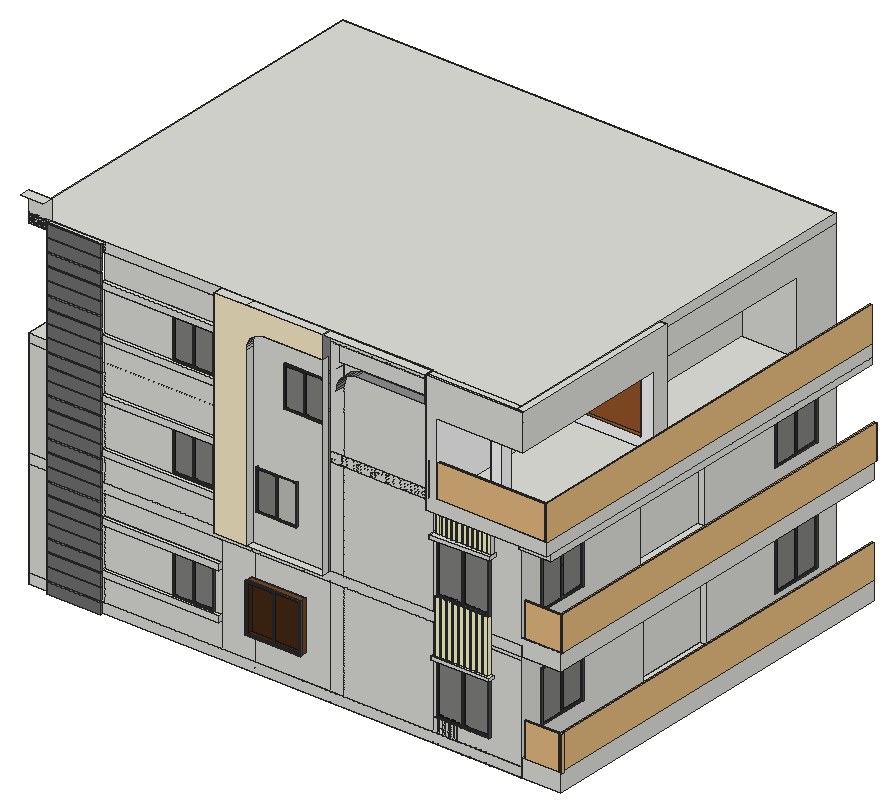
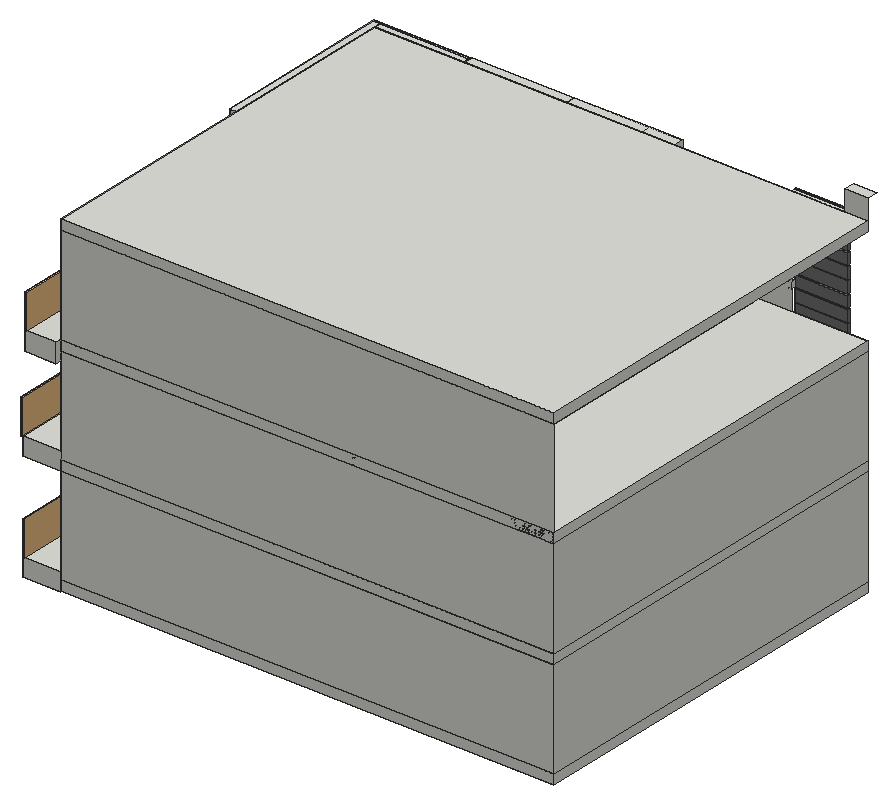
# SketchUp Ruby script. Lengths in inches.
U = 1.inch
M = Sketchup.active_model
def pt(a) = Geom::Point3d.new(a.map { |v| v * U })
def face(e, loops, mat)
  f = e.add_face(loops[0].map { |a| pt(a) })
  loops[1..].each { |l| e.add_face(l.map { |a| pt(a) }).erase! }
  f.material = f.back_material = mat if mat
  f
end
# faces: each face lists its corners as indices into pts; further lists are holes
def faces(e, pts, list, mat = nil) = list.each { |f| face(e, (f[0].is_a?(Array) ? f : [f]).map { |l| l.map { |i| pts[i] } }, mat) }
# xy, xz, yz: faces in a plane at the given z, y or x. An outline is a flat list of corners, or four numbers for a rectangle; further outlines are holes
def ring(l) = l.size == 4 ? [[l[0], l[1]], [l[2], l[1]], [l[2], l[3]], [l[0], l[3]]] : l.each_slice(2).to_a
def flat(e, list, mat, &to3) = list.each { |f| face(e, (f[0].is_a?(Array) ? f : [f]).map { |l| ring(l).map { |u, v| to3.(u, v) } }, mat) }
def xy(e, z, list, mat = nil) = flat(e, list, mat) { |x, y| [x, y, z] }
def xz(e, y, list, mat = nil) = flat(e, list, mat) { |x, z| [x, y, z] }
def yz(e, x, list, mat = nil) = flat(e, list, mat) { |y, z| [x, y, z] }
def lines(e, pts, list) = list.each { |a, b| e.add_line(pt(pts[a]), pt(pts[b])) }
# prism: a flat outline (further loops are holes) pulled along v
def prism(e, loops, v, mat = nil)
  f = face(e, loops, mat); d = Geom::Vector3d.new(v.map { |x| x * U })
  f.pushpull(f.normal.samedirection?(d) ? d.length : -d.length)
end
def box(e, o, s, mat = nil) = prism(e, [[o, [o[0] + s[0], o[1], o[2]], [o[0] + s[0], o[1] + s[1], o[2]], [o[0], o[1] + s[1], o[2]]]], [0, 0, s[2]], mat)
def at(x, y, z, deg = 0) = Geom::Transformation.translation(pt([x, y, z])) * Geom::Transformation.rotation(ORIGIN, Z_AXIS, deg.degrees)
def axes(o, x, y, z) = Geom::Transformation.new([*x, 0, *y, 0, *z, 0, *pt(o).to_a, 1])
def part(name) = M.definitions.add(name)
# library, detail: a bought-in or finely detailed component or shape, given as its bounding box
def library(name, o, s) = part(name).tap { |d| box(d.entities, o, s) }
def detail(e, o, s) = box(e.add_group.entities, o, s)
def put(e, d, t, mat = nil) = e.add_instance(d, t).tap { |i| i.material = mat if mat }
def group(e, t, mat = nil) = e.add_group.tap { |g| g.transformation = t; g.material = mat if mat }.entities
root = M.entities
M.materials.add("Glass_Tinted_Gray").color = [0, 0, 0]
M.materials["Glass_Tinted_Gray"].alpha = 0.125
M.materials.add("[0135_DarkGray]").color = [81, 81, 81]
M.materials.add("[Color D01]").color = [255, 242, 204]
M.materials.add("[Color E01]").color = [255, 255, 204]
M.materials.add("[Color M00]").color = [255, 255, 255]
M.materials.add("[Color M04]").color = [142, 142, 142]
M.materials.add("[Color M05]").color = [114, 114, 114]
M.materials.add("[Mirror 02]").color = [229, 229, 229]
M.materials.add("[Terrazzo Light Blue]").color = [196, 214, 227]
M.materials.add("[Wood Cherry Original]").color = [152, 86, 42]
M.materials.add("[Wood Veneer 01]").color = [120, 70, 37]
c1 = part("Group\#9")
box(c1.entities,[0,-2.75,0],[65.625,2.75,13.9375])
c2 = library("Wagner Glass Railing",[9.08,102.375,1.53],[2.51,145.5,42.05])
c3 = part("PENTEK_RP Fineline 50S_Sliding_DoorCase_E1")
box(c3.entities,[0,0,0],[1.51,3.66,99.27],"[0135_DarkGray]")
c4 = part("PENTEK_RP Fineline 50S_SlidingDooe_Case_E2")
box(c4.entities,[0,0,0],[96.25,3.66,1.51],"[0135_DarkGray]")
c5 = part("pentek_RP Fineline 50S_SlidingDoor_Case")
put(c5.entities,c3,at(97.76,0,0))
put(c5.entities,c4,at(1.51,0,0))
put(c5.entities,c3,at(0,0,0))
put(c5.entities,c4,at(1.51,0,97.76))
c6 = part("PENTEK_RP Fineline 50S_SlidingDoor_GlazingBead_2")
box(c6.entities,[0,0,0],[0.56,0.59,94.39],"[0135_DarkGray]")
c7 = part("PENTEK_RP Fineline 50S_SlidingDoor_Glass")
box(c7.entities,[0,0,0],[46.58,0.16,94.39],"Glass_Tinted_Gray")
c8 = part("PENTEK_RP Fineline 50S_SlidingDoor_GlazingBead")
box(c8.entities,[0,0,0],[45.47,0.59,0.56],"[0135_DarkGray]")
c9 = part("PENTEK_RP Fineline 50S_SlidingDoor_Leaf_E1")
xy(c9.entities,0,[[0,0,0.93,1.97],[0.93,1.57,1.49,1.97]],"[0135_DarkGray]")
xy(c9.entities,96.25,[[0,0,0.93,0,0.93,1.57,1.49,1.57,1.49,1.97,0,1.97]],"[0135_DarkGray]")
xz(c9.entities,0,[[0,0,0.93,96.25]],"[0135_DarkGray]")
xz(c9.entities,1.57,[[0.93,0,1.49,95.32],[0.93,95.32,1.49,96.25]],"[0135_DarkGray]")
xz(c9.entities,1.97,[[0,0,1.49,96.25]],"[0135_DarkGray]")
yz(c9.entities,0,[[0,0,1.97,96.25]],"[0135_DarkGray]")
yz(c9.entities,0.93,[[0,0,1.57,0.93],[0,0.93,1.57,95.32],[0,95.32,1.57,96.25]],"[0135_DarkGray]")
yz(c9.entities,1.49,[[1.57,0,1.97,95.32],[1.57,95.32,1.97,96.25]],"[0135_DarkGray]")
c10 = part("PENTEK_RP Fineline 50S_SlidingDoor_Leaf_E2")
xy(c10.entities,0,[[0,0,0,1.57,0.56,1.57,0.56,1.97,46.02,1.97,46.02,1.57,46.58,1.57,46.58,0]],"[0135_DarkGray]")
xy(c10.entities,0.93,[[0,0,46.58,1.57]],"[0135_DarkGray]")
xy(c10.entities,1.49,[[0.56,1.57,46.02,1.97]],"[0135_DarkGray]")
xz(c10.entities,0,[[0,0,46.58,0.93]],"[0135_DarkGray]")
xz(c10.entities,1.57,[[0,0,0.56,0.93],[46.02,0,46.58,0.93],[0.56,0.93,46.02,1.49]],"[0135_DarkGray]")
xz(c10.entities,1.97,[[0.56,0,46.02,1.49]],"[0135_DarkGray]")
yz(c10.entities,0,[[0,0,1.57,0.93]],"[0135_DarkGray]")
yz(c10.entities,0.56,[[1.57,0,1.97,0.93],[1.57,0.93,1.97,1.49]],"[0135_DarkGray]")
yz(c10.entities,46.02,[[1.57,0,1.97,0.93],[1.57,0.93,1.97,1.49]],"[0135_DarkGray]")
yz(c10.entities,46.58,[[0,0,1.57,0.93]],"[0135_DarkGray]")
c11 = part("PENTEK_RP Fineline S_SlidingDoor_Leaf1")
put(c11.entities,c6,at(0.93,0,0.93))
put(c11.entities,c6,at(46.96,0,0.93))
put(c11.entities,c7,at(1.49,1.42,0.93))
put(c11.entities,c8,at(1.49,0,0.93))
put(c11.entities,c7,at(1.49,0.59,0.93),"[Terrazzo Light Blue]")
put(c11.entities,c9,at(0,0,0))
put(c11.entities,c9,axes([48.44,0,0],[-1,0,0],[0,1,0],[0,0,1]))
put(c11.entities,c10,axes([0.93,0,96.25],[1,0,0],[0,1,0],[0,0,-1]))
put(c11.entities,c10,at(0.93,0,0))
put(c11.entities,c8,at(1.49,0,94.77))
c12 = part("PENTEK_RP Fineline 50S_SlidingDoor_Leaf2")
put(c12.entities,c7,at(1.49,1.42,0.93))
put(c12.entities,c8,at(1.49,0,94.77))
put(c12.entities,c6,at(46.96,0,0.93))
put(c12.entities,c7,at(1.49,0.59,0.93),"[Mirror 02]")
put(c12.entities,c6,at(0.93,0,0.93))
put(c12.entities,c9,at(0,0,0))
put(c12.entities,c9,axes([48.44,0,0],[-1,0,0],[0,1,0],[0,0,1]))
put(c12.entities,c8,at(1.49,0,0.93))
put(c12.entities,c10,axes([0.93,0,96.25],[1,0,0],[0,1,0],[0,0,-1]))
put(c12.entities,c10,at(0.93,0,0))
c13 = part("PENTEK - Slimmest Steel Sliding Door / Window\#1")
put(c13.entities,c5,at(0,-1.88,-0.09))
put(c13.entities,c11,at(1.51,-2.27,1.42))
put(c13.entities,c12,at(49.32,-0.3,1.42))
c14 = part("Group\#10")
box(c14.entities,[-76.71,-4.875,-2.4375],[142.83,4.875,7.6875])
prism(root,[[[538.49,59.34,350.59],[610.93,62.6,350.59],[611.36,53.02,350.59],[538.92,49.75,350.59]]],[0,0,4.15])
xy(root,119.69,[[643.25,62.39,690.1875,542.39]])
xy(root,120,[[[39.25,62.39,643.25,542.39],[172.25,71.39,634.25,533.39]]])
xy(root,132,[[[39.25,62.39,643.25,542.39],[172.25,71.39,634.25,533.39]],[172.25,71.39,634.25,533.39]])
xy(root,141.25,[[643.25,62.39,690.1875,542.39],[634.375,246.18,643.25,344.71]])
xy(root,152.27,[[540.39,57.14,545.76,62.39],[546.71,57.14,552.08,62.39],[553.03,57.14,558.4,62.39],[559.28,57.14,564.65,62.39],[565.65,57.14,571.03,62.39],
  [572.84,57.14,578.21,62.39],[579.65,57.14,585.03,62.39],[586.71,57.14,592.09,62.39],[592.73,57.14,598.11,62.39],[599.11,57.14,606.05,62.39]])
xy(root,165.75,[[313.83,50.27,379.89,59.77]],"[Wood Veneer 01]")
xy(root,216.35,[[538.15,53.52,608.9,62.39]])
xy(root,218.67,[[548.22,57.14,554.35,62.39],[555.28,57.14,561.41,62.39]])
xy(root,219.92,[[538.15,53.52,608.9,53.52,608.9,62.39,561.41,62.39,561.41,57.14,555.28,57.14,555.28,62.39,554.35,62.39,554.35,57.14,548.22,57.14,548.22,62.39,547.1,62.39,547.1,57.14,540.97,57.14,540.97,62.39,538.15,62.39]])
xy(root,225.5,[[313.83,50.27,379.89,59.77]],"[Wood Veneer 01]")
xy(root,252,[[[39.25,62.39,643.25,62.39,643.25,246.18,634.375,246.18,634.375,344.71,643.25,344.71,643.25,542.39,39.25,542.39],[172.25,71.39,634.25,533.39]],[643.25,62.39,643.25,246.18,634.375,246.18,634.375,344.71,643.25,344.71,643.25,542.39,690.1875,542.39,690.1875,62.39]])
xy(root,264,[[275.5,50.27,315.25,62.39],[315.25,50.27,408.24,59.45],[315.25,59.45,408.24,62.39],[172.25,71.39,634.25,533.39]])
xy(root,273.5625,[[643.25,62.39,690.1875,62.39,690.1875,542.39,643.25,542.39,643.25,341.58,634.375,341.58,634.375,242.52,643.25,242.52]])
xy(root,285.55,[[598.15,57.66,604.28,62.91]])
xy(root,285.71,[[540.97,57.14,547.1,62.39],[548.22,57.14,554.35,62.39],[555.28,57.14,561.41,62.39]])
xy(root,285.87,[[562.53,57.66,568.65,62.91],[569.46,57.66,575.59,62.91],[576.53,57.66,582.65,62.91],[584.03,57.66,590.15,62.91],[591.28,57.66,597.4,62.91]])
xy(root,351.625,[[541.21,57.14,546.27,62.39]])
xy(root,372.625,[[643.25,57.6,681.9,549.14],[634.375,242.52,643.25,272.93],[634.375,272.93,643.25,341.58]])
xy(root,379.8125,[[534.125,51.64,534.125,57.14,539.4375,57.14,539.4375,62.39,541.21,62.39,541.21,57.14,547.02,57.14,547.02,62.39,548.46,62.39,548.46,57.14,553.52,57.14,553.52,62.39,555.16,62.39,555.16,57.14,560.23,57.14,560.23,62.39,561.35,62.39,561.35,57.14,566.41,57.14,566.41,62.39,567.85,62.39,567.85,57.14,572.91,57.14,572.91,62.39,574.79,62.39,574.79,57.14,579.85,57.14,579.85,62.39,580.73,62.39,580.73,57.14,585.79,57.14,585.79,62.39,586.85,62.39,586.85,57.14,591.91,57.14,591.91,62.39,592.54,62.39,592.54,57.14,597.6,57.14,597.6,62.39,598.48,62.39,598.48,57.14,603.54,57.14,603.54,62.39,603.5625,62.39,603.5625,57.14,608.625,57.14,608.625,62.39,643.25,62.39,643.25,57.6,681.9,57.6,681.9,51.64],[534.125,57.14,539.4375,62.39],[541.21,57.14,546.27,62.39],[546.27,57.14,547.02,62.39],[548.46,57.14,553.52,62.39],
  [555.16,57.14,560.23,62.39],[561.35,57.14,566.41,62.39],[567.85,57.14,572.91,62.39],[574.79,57.14,579.85,62.39],[580.73,57.14,585.79,62.39],
  [586.85,57.14,591.91,62.39],[592.54,57.14,597.6,62.39],[598.48,57.14,603.54,62.39],[603.5625,57.14,608.625,62.39]])
xy(root,384,[[547.02,62.39,643.25,62.39,643.25,482.24,634.25,482.24,634.25,71.39,547.02,71.39]])
xy(root,396,[[547.02,51.64,681.9,51.64,681.9,272.93,652.0625,272.93,652.0625,252.8,643.25,252.8,643.25,62.39,547.02,62.39],[172.25,71.39,547.02,71.39,547.02,252.8,634.25,252.8,634.25,272.93,575.75,272.93,575.75,482.24,634.25,482.24,634.25,533.39,172.25,533.39],[634.25,252.8,643.25,272.93],[643.25,272.93,681.9,549.14]])
xy(root,396,[[592.44,78.38,605,93.32]],"[Wood Cherry Original]")
xy(root,407.63,[[565.8,252.8,635.55,258.68]],"[Wood Cherry Original]")
xy(root,470.57,[[565.8,252.8,635.55,258.68]],"[Wood Cherry Original]")
xy(root,480.375,[[[556.7,64.84,639.52,239.78],[592.44,78.38,605,93.32]],[584.07,281.12,632.51,473.74]],"[Wood Cherry Original]")
xy(root,484.0625,[[[547.02,51.64,652.0625,252.8],[556.7,64.84,639.52,239.78]],[[575.75,272.93,643.25,482.24],[584.07,281.12,632.51,473.74]]])
xy(root,496.9375,[[425.1875,62.39,449.88,64.02]])
xy(root,496.9375,[[449.88,50.27,533.5,62.39]],"[Color M04]")
xy(root,501.33,[[337.14,50.27,408.24,59.45]])
xy(root,516,[[[39.25,62.39,643.25,542.39],[172.25,71.39,634.25,533.39]]])
xy(root,528,[[275.5,50.27,315.25,62.39],[315.25,50.27,408.24,62.39],[408.24,50.27,533.5,62.39],[534.125,51.64,652.0625,53.64],[534.125,53.64,643.25,62.39],
  [643.25,53.64,652.0625,272.93],[67.04,57.77,132.66,62.39]])
xy(root,552.6875,[[39.25,49.27,67.04,62.39]])
xz(root,50.27,[[275.5,264,315.25,264,315.25,479.4375,315.4375,482.29,315.99,485.1,316.92,487.8125,318.18,490.38,319.77,492.76,321.66,494.92,323.8125,496.8,326.19,498.39,328.76,499.66,331.47,500.58,334.28,501.14,337.14,501.33,408.24,501.33,408.24,528,275.5,528]],"[Color D01]")
xz(root,51.64,[[534.125,379.8125,681.9,379.8125,681.9,396,547.02,396,547.02,484.0625,652.0625,484.0625,652.0625,528,534.125,528]])
xz(root,53.52,[[538.15,216.35,608.9,219.92]])
xz(root,57.14,[[548.22,218.67,554.35,219.92],[555.28,218.67,561.41,219.92]])
xz(root,57.14,[[540.97,219.92,547.1,285.71],[548.22,219.92,554.35,285.71],[555.28,219.92,561.41,285.71],[541.21,351.625,546.27,379.8125],[548.46,351.625,553.52,379.8125],
  [555.16,351.625,560.23,379.8125],[561.35,351.625,566.41,379.8125],[567.85,351.625,572.91,379.8125],[574.79,351.625,579.85,379.8125],[580.73,351.625,585.79,379.8125],
  [586.85,351.625,591.91,379.8125],[592.54,351.625,597.6,379.8125],[598.48,351.625,603.54,379.8125],[603.5625,351.625,608.625,379.8125]],"[Color E01]")
xz(root,57.6,[[643.25,372.625,681.9,379.8125]])
xz(root,57.66,[[562.53,216.45,568.65,285.87],[569.46,216.45,575.59,285.87],[576.53,216.45,582.65,285.87],[584.03,216.45,590.15,285.87],[591.28,216.45,597.4,285.87],
  [598.15,216.45,604.28,285.55]],"[Color E01]")
xz(root,59.45,[[315.25,264,408.24,264,408.24,501.33,337.14,501.33,334.28,501.14,331.47,500.58,328.76,499.66,326.19,498.39,323.8125,496.8,321.66,494.92,319.77,492.76,318.18,490.38,316.92,487.8125,315.99,485.1,315.4375,482.29,315.25,479.4375]])
xz(root,59.77,[[313.83,165.75,379.89,225.5]],"[Wood Veneer 01]")
xz(root,62.39,[[599.11,119.69,606.05,119.69,606.05,132,643.25,132,643.25,247.5,554.35,247.5,554.35,219.92,555.28,219.92,555.28,218.67,561.41,218.67,561.41,219.92,608.9,219.92,608.9,216.35,539.4375,216.35,539.4375,132,540.39,132,540.39,131.69,540.97,131.69,540.97,132,540.39,132,540.39,152.27,540.97,152.27,540.97,153.4,547.1,153.4,547.1,152.27,548.22,152.27,548.22,153.4,554.35,153.4,554.35,152.27,555.28,152.27,555.28,153.4,561.41,153.4,561.41,152.27,564.65,152.27,564.65,120,599.11,120],[561.41,119.69,564.65,120],[564.65,119.69,565.65,120],[565.65,119.69,571.03,120],[571.03,119.69,572.84,120],
  [572.84,119.69,578.21,120],[578.21,119.69,579.65,120],[579.65,119.69,585.03,120],[585.03,119.69,586.71,120],[586.71,119.69,592.09,120],
  [592.09,119.69,592.73,120],[592.73,119.69,598.11,120],[598.11,119.69,599.11,120],[599.11,119.69,606.05,120],[606.05,119.69,643.25,120],
  [643.25,119.69,690.1875,119.69,690.1875,141.25,643.25,141.25,643.25,132,606.05,132,606.05,120,643.25,120],[39.25,120,67.04,132],[67.04,120,132.66,132],[275.5,120,315.25,132],[315.25,120,408.24,132],
  [408.24,120,425.1875,132],[534.125,120,539.4375,132],[540.39,120,540.39,131.69,540.97,131.69,540.97,132,545.76,132,545.76,120],[561.41,120,564.65,132],[604.48,120,606.05,132],
  [539.4375,131.69,540.39,132],[547.1,131.69,548.22,132],[554.35,131.69,555.28,132],[39.25,132,67.04,252],[67.04,132,132.66,252],
  [132.66,132,275.5,252],[275.5,132,315.25,252],[315.25,132,408.24,252],[408.24,132,425.1875,252],[425.1875,132,534.125,252],
  [534.125,132,539.4375,132,539.4375,216.35,538.15,216.35,538.15,219.92,539.4375,219.92,539.4375,252,534.125,252],[539.4375,132,540.39,132,540.39,152.27,540.97,152.27,540.97,153.4,547.1,153.4,547.1,152.27,548.22,152.27,548.22,153.4,554.35,153.4,554.35,152.27,555.28,152.27,555.28,153.4,561.41,153.4,561.41,152.27,564.65,152.27,564.65,132,565.65,132,565.65,152.27,571.03,152.27,571.03,132,572.84,132,572.84,152.27,578.21,152.27,578.21,132,579.65,132,579.65,152.27,585.03,152.27,585.03,132,586.71,132,586.71,152.27,592.09,152.27,592.09,132,592.73,132,592.73,152.27,598.11,152.27,598.11,132,599.11,132,599.11,152.27,606.05,152.27,606.05,132,643.25,132,643.25,247.5,561.41,247.5,561.41,219.92,608.9,219.92,608.9,216.35,539.4375,216.35],[540.39,132,540.97,152.27],[545.76,132,546.71,132,546.71,152.27,547.1,152.27,547.1,153.4,540.97,153.4,540.97,152.27,545.76,152.27],[546.71,132,547.1,152.27],
  [547.1,132,548.22,152.27],[548.22,132,552.08,152.27],[552.08,132,553.03,132,553.03,152.27,554.35,152.27,554.35,153.4,548.22,153.4,548.22,152.27,552.08,152.27],[553.03,132,554.35,152.27],[554.35,132,555.28,152.27],
  [555.28,132,558.4,152.27],[558.4,132,559.28,132,559.28,152.27,561.41,152.27,561.41,153.4,555.28,153.4,555.28,152.27,558.4,152.27],[559.28,132,561.41,152.27],[561.41,132,564.65,152.27],[565.65,132,571.03,152.27],
  [572.84,132,578.21,152.27],[579.65,132,585.03,152.27],[586.71,132,592.09,152.27],[592.73,132,598.11,152.27],[599.11,132,606.05,152.27],
  [538.15,216.35,539.4375,219.92],[539.4375,216.35,608.9,216.35,608.9,219.92,561.41,219.92,561.41,218.67,555.28,218.67,555.28,219.92,554.35,219.92,554.35,218.67,548.22,218.67,548.22,219.92,547.1,219.92,547.1,218.67,540.97,218.67,540.97,219.92,539.4375,219.92],[540.97,218.67,547.1,218.67,547.1,247.5,546.27,247.5,546.27,219.32,541.21,219.32,541.21,247.5,540.97,247.5],[548.22,218.67,554.35,247.5],[555.28,218.67,561.41,247.5],
  [541.21,219.32,546.27,219.32,546.27,247.5,547.1,247.5,547.1,252,540.97,252,540.97,247.5,541.21,247.5],[539.4375,219.92,540.97,247.5],[547.1,219.92,548.22,247.5],[554.35,219.92,555.28,247.5],[539.4375,247.5,540.97,252],
  [547.1,247.5,548.22,252],[548.22,247.5,554.35,252],[554.35,247.5,555.28,252],[555.28,247.5,561.41,252],[561.41,247.5,643.25,252],
  [39.25,252,67.04,264],[67.04,252,132.66,264],[275.5,252,315.25,264],[315.25,252,408.24,264],[408.24,252,425.1875,264],
  [534.125,252,539.4375,264],[561.41,252,690.1875,252,690.1875,273.5625,643.25,273.5625,643.25,379.8125,546.27,379.8125,546.27,351.625,541.21,351.625,541.21,379.8125,539.4375,379.8125,539.4375,264,540.97,264,540.97,285.71,547.1,285.71,547.1,264,548.22,264,548.22,285.71,554.35,285.71,554.35,264,555.28,264,555.28,285.71,561.41,285.71],[540.97,252,547.1,259.125],[540.97,259.125,547.1,264],[39.25,264,67.04,384],
  [67.04,264,132.66,384],[132.66,264,275.5,264,275.5,481.34,209.375,481.34,209.375,486.59,275.5,486.59,275.5,516,132.66,516],[275.5,264,315.25,384],[315.25,264,408.24,384],[408.24,264,425.1875,384],
  [425.1875,264,534.125,384],[548.22,264,554.35,285.71],[555.28,264,561.41,285.71],[534.125,379.8125,547.02,384],[547.02,379.8125,643.25,384],
  [275.5,384,315.25,516],[315.25,384,408.24,516],[408.24,384,425.1875,384,425.1875,496.9375,418.125,496.9375,418.125,516,408.24,516],[425.1875,384,534.125,384,534.125,516,533.5,516,533.5,496.9375,533.61,496.9375,533.61,471.875,532.42,471.875,532.42,496.9375,425.1875,496.9375],[547.02,384,643.25,396],
  [418.125,496.9375,533.5,516],[39.25,516,67.04,552.6875],[67.04,516,132.66,528],[275.5,516,315.25,528],[315.25,516,408.24,528],
  [408.24,516,533.5,528],[534.125,516,643.25,528]])
xz(root,64.02,[[425.1875,472.24,425.1875,496.9375,449.88,496.9375,446.66,496.73,443.49,496.1,440.43,495.06,437.53,493.63,434.85,491.83,432.42,489.71,430.29,487.28,428.5,484.59,427.07,481.69,426.03,478.64,425.4,475.47]])
xz(root,64.84,[[556.7,480.375,639.52,484.0625]],"[Wood Cherry Original]")
xz(root,71.39,[[172.25,132,634.25,252],[172.25,264,634.25,384],[172.25,384,547.02,396]])
xz(root,78.38,[[592.44,396,605,480.375]],"[Color M00]")
xz(root,93.32,[[592.44,396,605,480.375]],"[Color M00]")
xz(root,239.78,[[556.7,480.375,639.52,484.0625]],"[Wood Cherry Original]")
xz(root,242.52,[[634.375,273.5625,643.25,372.625]])
xz(root,246.18,[[634.375,141.25,643.25,252]])
xz(root,252.8,[[[547.02,396,652.0625,484.0625],[565.8,407.63,635.55,470.57]]],"[Color M00]")
xz(root,258.68,[[565.8,407.63,635.55,470.57]],"[Wood Cherry Original]")
xz(root,272.93,[[575.75,396,643.25,484.0625],[643.25,396,652.0625,528]])
xz(root,281.12,[[584.07,480.375,632.51,484.0625]],"[Wood Cherry Original]")
xz(root,341.58,[[634.375,273.5625,643.25,372.625]])
xz(root,344.71,[[634.375,141.25,643.25,252]])
xz(root,473.74,[[584.07,480.375,632.51,484.0625]],"[Wood Cherry Original]")
xz(root,482.24,[[634.25,384,643.25,384,643.25,484.0625,575.75,484.0625,575.75,396,634.25,396]])
xz(root,533.39,[[172.25,132,634.25,252],[172.25,264,634.25,384],[172.25,384,634.25,396],[172.25,396,634.25,516]])
xz(root,542.39,[[643.25,119.69,690.1875,141.25],[39.25,132,643.25,252],[643.25,252,690.1875,273.5625],[39.25,264,643.25,384],[39.25,384,643.25,516]])
xz(root,549.14,[[643.25,372.625,681.9,396]])
yz(root,39.25,[[62.39,132,542.39,252],[62.39,264,542.39,384]])
yz(root,172.25,[[71.39,132,533.39,252],[71.39,264,533.39,384],[71.39,384,533.39,396],[71.39,396,533.39,516]])
yz(root,275.5,[[50.27,264,62.39,528]])
yz(root,313.83,[[50.27,165.75,59.77,225.5]],"[Wood Veneer 01]")
yz(root,315.25,[[50.27,264,59.45,479.4375]])
yz(root,379.89,[[50.27,165.75,59.77,225.5]],"[Wood Veneer 01]")
yz(root,408.24,[[50.27,264,59.45,501.33]])
yz(root,408.24,[[59.45,264,59.45,501.33,50.27,501.33,50.27,528,62.39,528,62.39,264]],"[Color M04]")
yz(root,425.1875,[[62.39,472.24,64.02,496.9375]])
yz(root,533.5,[[50.27,496.9375,62.39,528]],"[Color M04]")
yz(root,534.125,[[51.64,379.8125,62.39,516],[51.64,516,53.64,528],[53.64,516,62.39,528]])
yz(root,538.15,[[53.52,216.35,62.39,219.92]])
yz(root,540.97,[[57.14,219.92,62.39,285.71]])
yz(root,541.21,[[57.14,351.625,62.39,379.8125]],"[Color E01]")
yz(root,546.27,[[57.14,351.625,62.39,379.8125]],"[Color E01]")
yz(root,547.02,[[62.39,384,62.39,396,51.64,396,51.64,484.0625,252.8,484.0625,252.8,396,71.39,396,71.39,384]],"[Color M00]")
yz(root,547.1,[[57.14,219.92,62.39,285.71]],"[Color E01]")
yz(root,548.22,[[57.14,218.67,62.39,219.92],[57.14,219.92,62.39,285.71]])
yz(root,548.46,[[57.14,351.625,62.39,379.8125]],"[Color E01]")
yz(root,553.52,[[57.14,351.625,62.39,379.8125]],"[Color E01]")
yz(root,554.35,[[57.14,218.67,62.39,219.92]])
yz(root,554.35,[[57.14,219.92,62.39,285.71]],"[Color E01]")
yz(root,555.16,[[57.14,351.625,62.39,379.8125]],"[Color E01]")
yz(root,555.28,[[57.14,218.67,62.39,219.92],[57.14,219.92,62.39,285.71]])
yz(root,556.7,[[64.84,480.375,239.78,484.0625]],"[Wood Cherry Original]")
yz(root,560.23,[[57.14,351.625,62.39,379.8125]],"[Color E01]")
yz(root,561.35,[[57.14,351.625,62.39,379.8125]],"[Color E01]")
yz(root,561.41,[[57.14,218.67,62.39,219.92]])
yz(root,561.41,[[57.14,219.92,62.39,285.71]],"[Color E01]")
yz(root,562.53,[[57.66,216.45,62.91,285.87]])
yz(root,565.8,[[252.8,407.63,258.68,470.57]],"[Wood Cherry Original]")
yz(root,566.41,[[57.14,351.625,62.39,379.8125]],"[Color E01]")
yz(root,567.85,[[57.14,351.625,62.39,379.8125]],"[Color E01]")
yz(root,568.65,[[57.66,216.45,62.91,285.87]])
yz(root,569.46,[[57.66,216.45,62.91,285.87]])
yz(root,572.91,[[57.14,351.625,62.39,379.8125]],"[Color E01]")
yz(root,574.79,[[57.14,351.625,62.39,379.8125]],"[Color E01]")
yz(root,575.59,[[57.66,216.45,62.91,285.87]],"[Color E01]")
yz(root,575.75,[[272.93,396,482.24,484.0625]])
yz(root,576.53,[[57.66,216.45,62.91,285.87]])
yz(root,579.85,[[57.14,351.625,62.39,379.8125]],"[Color E01]")
yz(root,580.73,[[57.14,351.625,62.39,379.8125]],"[Color E01]")
yz(root,582.65,[[57.66,216.45,62.91,285.87]],"[Color E01]")
yz(root,584.03,[[57.66,216.45,62.91,285.87]])
yz(root,584.07,[[281.12,480.375,473.74,484.0625]])
yz(root,585.79,[[57.14,351.625,62.39,379.8125]],"[Color E01]")
yz(root,586.85,[[57.14,351.625,62.39,379.8125]],"[Color E01]")
yz(root,590.15,[[57.66,216.45,62.91,285.87]],"[Color E01]")
yz(root,591.28,[[57.66,216.45,62.91,285.87]])
yz(root,591.91,[[57.14,351.625,62.39,379.8125]],"[Color E01]")
yz(root,592.44,[[78.38,396,93.32,480.375]],"[Color M00]")
yz(root,592.54,[[57.14,351.625,62.39,379.8125]])
yz(root,597.4,[[57.66,216.45,62.91,285.87]],"[Color E01]")
yz(root,597.6,[[57.14,351.625,62.39,379.8125]],"[Color E01]")
yz(root,598.15,[[57.66,216.45,62.91,285.55]])
yz(root,598.48,[[57.14,351.625,62.39,379.8125]],"[Color E01]")
yz(root,603.54,[[57.14,351.625,62.39,379.8125]])
yz(root,603.5625,[[57.14,351.625,62.39,379.8125]])
yz(root,604.28,[[57.66,216.45,62.91,285.55]],"[Color E01]")
yz(root,605,[[78.38,396,93.32,480.375]],"[Color M00]")
yz(root,608.625,[[57.14,351.625,62.39,379.8125]])
yz(root,608.9,[[53.52,216.35,62.39,219.92]])
yz(root,632.51,[[281.12,480.375,473.74,484.0625]],"[Wood Cherry Original]")
yz(root,634.25,[[71.39,132,533.39,252],[71.39,264,533.39,384],[482.24,384,533.39,396]])
yz(root,634.375,[[246.18,141.25,344.71,252],[242.52,273.5625,341.58,372.625]])
yz(root,635.55,[[252.8,407.63,258.68,470.57]],"[Wood Cherry Original]")
yz(root,639.52,[[64.84,480.375,239.78,484.0625]],"[Wood Cherry Original]")
yz(root,643.25,[[62.39,119.69,542.39,120],[62.39,132,542.39,141.25],[62.39,141.25,246.18,252],[344.71,141.25,542.39,252],[62.39,273.5625,242.52,372.625],
  [341.58,273.5625,542.39,372.625],[57.6,372.625,62.39,379.8125],[62.39,372.625,272.93,384],[272.93,372.625,542.39,384],[542.39,372.625,549.14,396],
  [62.39,384,272.93,396],[272.93,384,482.24,396],[482.24,384,542.39,396],[482.24,396,542.39,396,542.39,516,272.93,516,272.93,484.0625,482.24,484.0625],[53.64,516,62.39,528],
  [62.39,516,272.93,528]])
yz(root,652.0625,[[252.8,396,272.93,396,272.93,528,51.64,528,51.64,484.0625,252.8,484.0625]])
yz(root,681.9,[[57.6,372.625,549.14,379.8125],[51.64,379.8125,549.14,396]])
yz(root,690.1875,[[62.39,119.69,542.39,141.25],[62.39,252,542.39,273.5625]])
p = [[425.4,50.27,475.47],[425.1875,50.27,472.24],[425.1875,62.39,472.24],[425.1875,64.02,472.24],[425.4,64.02,475.47],[426.03,50.27,478.64],
  [426.03,64.02,478.64],[427.07,50.27,481.69],[427.07,64.02,481.69],[315.4375,50.27,482.29],[315.25,50.27,479.4375],[315.25,59.45,479.4375],
  [315.4375,59.45,482.29],[428.5,50.27,484.59],[428.5,64.02,484.59],[315.99,50.27,485.1],[315.99,59.45,485.1],[430.29,50.27,487.28],
  [430.29,64.02,487.28],[316.92,50.27,487.8125],[316.92,59.45,487.8125],[432.42,50.27,489.71],[432.42,64.02,489.71],[318.18,50.27,490.38],
  [318.18,59.45,490.38],[434.85,50.27,491.83],[434.85,64.02,491.83],[319.77,50.27,492.76],[319.77,59.45,492.76],[437.53,50.27,493.63],
  [437.53,64.02,493.63],[321.66,50.27,494.92],[321.66,59.45,494.92],[440.43,50.27,495.06],[440.43,64.02,495.06],[323.8125,50.27,496.8],
  [323.8125,59.45,496.8],[443.49,50.27,496.1],[443.49,64.02,496.1],[446.66,50.27,496.73],[446.66,64.02,496.73],[449.88,50.27,496.9375],
  [449.88,64.02,496.9375],[449.88,62.39,496.9375],[326.19,50.27,498.39],[326.19,59.45,498.39],[328.76,50.27,499.66],[328.76,59.45,499.66],
  [331.47,50.27,500.58],[331.47,59.45,500.58],[334.28,50.27,501.14],[334.28,59.45,501.14],[337.14,50.27,501.33],[337.14,59.45,501.33],
  [425.1875,50.27,496.9375],[425.1875,62.39,496.9375],[634.25,71.39,484.0625],[634.25,71.39,516],[643.25,252.8,484.0625],[643.25,272.93,484.0625],
  [643.25,53.64,516],[643.25,53.64,484.0625],[652.0625,53.64,516]]
faces(root,p,[[0,1,2,3,4],[5,0,4,6],[7,5,6,8],[13,7,8,14],[17,13,14,18],[21,17,18,22],[25,21,22,26],[29,25,26,30],
  [33,29,30,34],[37,33,34,38],[39,37,38,40],[41,39,40,42,43]],"[Color M04]")
faces(root,p,[[9,10,11,12],[15,9,12,16],[19,15,16,20],[23,19,20,24],[27,23,24,28],[31,27,28,32],[35,31,32,36],[44,35,36,45],
  [46,44,45,47],[48,46,47,49],[50,48,49,51],[52,50,51,53]])
lines(root,p,[[54,55],[56,57],[58,59],[60,61],[60,62]])
g1 = group(root,at(163.25,542.39,120))
box(g1,[-124,-480,0],[604,480,12])
put(root,c1,at(67.04,57.77,121.875),"[Color M05]")
put(root,c1,at(67.04,57.77,137.5625),"[Color M05]")
put(root,c2,axes([612.93,74.81,139.21],[0,-1,0],[0.3167,0,0],[0,0,1]))
put(root,c2,axes([678.59,-275.34,139.72],[1,0,0],[0,3.29897,0],[0,0,1]))
put(root,c13,axes([542.36,58.36,152.33],[0.6478,0,0],[0,0.6478,0],[0,0,0.6478]))
put(root,c13,axes([644.07,447.53,152.92],[0,0.6478,0],[-0.6478,0,0],[0,0,0.6478]))
put(root,c1,at(67.04,57.77,153.25),"[Color M05]")
put(root,c14,at(209.375,62.39,164.9375))
put(root,c13,axes([644.07,89.22,164.79],[0,0.6478,0],[-0.6478,0,0],[0,0,0.6478]))
put(root,c13,axes([315.02,50.42,166.72],[0.68057,0,0],[0,0.5,0],[0,0,0.605]))
put(root,c1,at(67.04,57.77,168.9375),"[Color M05]")
put(root,c13,axes([217.18,61.75,170.23],[0.5,0,0],[0,0.5,0],[0,0,0.5]))
put(root,c1,at(67.04,57.77,184.625),"[Color M05]")
put(root,c1,at(67.04,57.77,200.3125),"[Color M05]")
put(root,c1,at(67.04,57.77,216),"[Color M05]")
put(root,c14,at(209.375,61.89,222.54))
put(root,c1,at(67.04,57.77,231.6875),"[Color M05]")
put(root,c1,at(67.04,57.77,247.375),"[Color M05]")
g2 = group(root,at(163.25,542.39,252))
box(g2,[-124,-480,0],[604,480,12])
put(root,c1,at(67.04,57.77,263.0625),"[Color M05]")
put(root,c2,axes([612.93,74.81,270.28],[0,-1,0],[0.3167,0,0],[0,0,1]))
put(root,c2,axes([681.11,-275.34,272.03],[1,0,0],[0,3.29897,0],[0,0,1]))
put(root,c1,at(67.04,57.77,278.75),"[Color M05]")
put(root,c13,axes([542.36,58.36,285.77],[0.6478,0,0],[0,0.6478,0],[0,0,0.6478]))
put(root,c13,axes([644.07,89.22,289.79],[0,0.6478,0],[-0.6478,0,0],[0,0,0.6478]))
put(root,c13,axes([644.07,447.53,290.86],[0,0.6478,0],[-0.6478,0,0],[0,0,0.6478]))
put(root,c1,at(67.04,57.77,294.4375),"[Color M05]")
put(root,c14,at(209.375,62.39,297.91))
put(root,c13,axes([320.66,59.31,299.59],[0.5,0,0],[0,0.5,0],[0,0,0.5]))
put(root,c13,axes([217.18,61.75,305.48],[0.5,0,0],[0,0.5,0],[0,0,0.5]))
put(root,c1,at(67.04,57.77,310.125),"[Color M05]")
put(root,c1,at(67.04,57.77,325.8125),"[Color M05]")
put(root,c1,at(67.04,57.77,341.5),"[Color M05]")
put(root,c14,at(209.375,62.39,357.57))
put(root,c1,at(67.04,57.77,357.1875),"[Color M05]")
put(root,c1,at(67.04,57.77,372.875),"[Color M05]")
g3 = group(root,at(163.25,542.39,384))
box(g3,[-124,-480,0],[604,480,12])
put(root,c1,at(67.04,57.77,388.5625),"[Color M05]")
put(root,c2,axes([435.82,64.09,392.77],[0,-1,0],[0.98969,0,0],[0,0,1]))
put(root,c2,axes([670.3125,-298.4,394.47],[1,0,0],[0,3.41924,0],[0,0,1]))
put(root,c1,at(67.04,57.77,404.25),"[Color M05]")
put(root,c1,at(67.04,57.77,419.9375),"[Color M05]")
put(root,c14,at(209.375,62.39,423.03))
put(root,c13,axes([358.58,54.14,428.49],[0.5,0,0],[0,0.5,0],[0,0,0.5]))
put(root,c13,axes([217.18,61.75,428.67],[0.5,0,0],[0,0.5,0],[0,0,0.5]))
put(root,c1,at(67.04,57.77,435.625),"[Color M05]")
put(root,c1,at(67.04,57.77,451.3125),"[Color M05]")
put(root,c1,at(67.04,57.77,467),"[Color M05]")
put(root,c14,at(209.375,62.39,481.34))
put(root,c1,at(67.04,57.77,482.6875),"[Color M05]")
put(root,c1,at(67.04,57.77,498.375),"[Color M05]")
put(root,c1,at(67.04,57.77,514.0625),"[Color M05]")
g4 = group(root,at(163.25,542.39,516))
box(g4,[-124,-480,0],[604,480,12])
